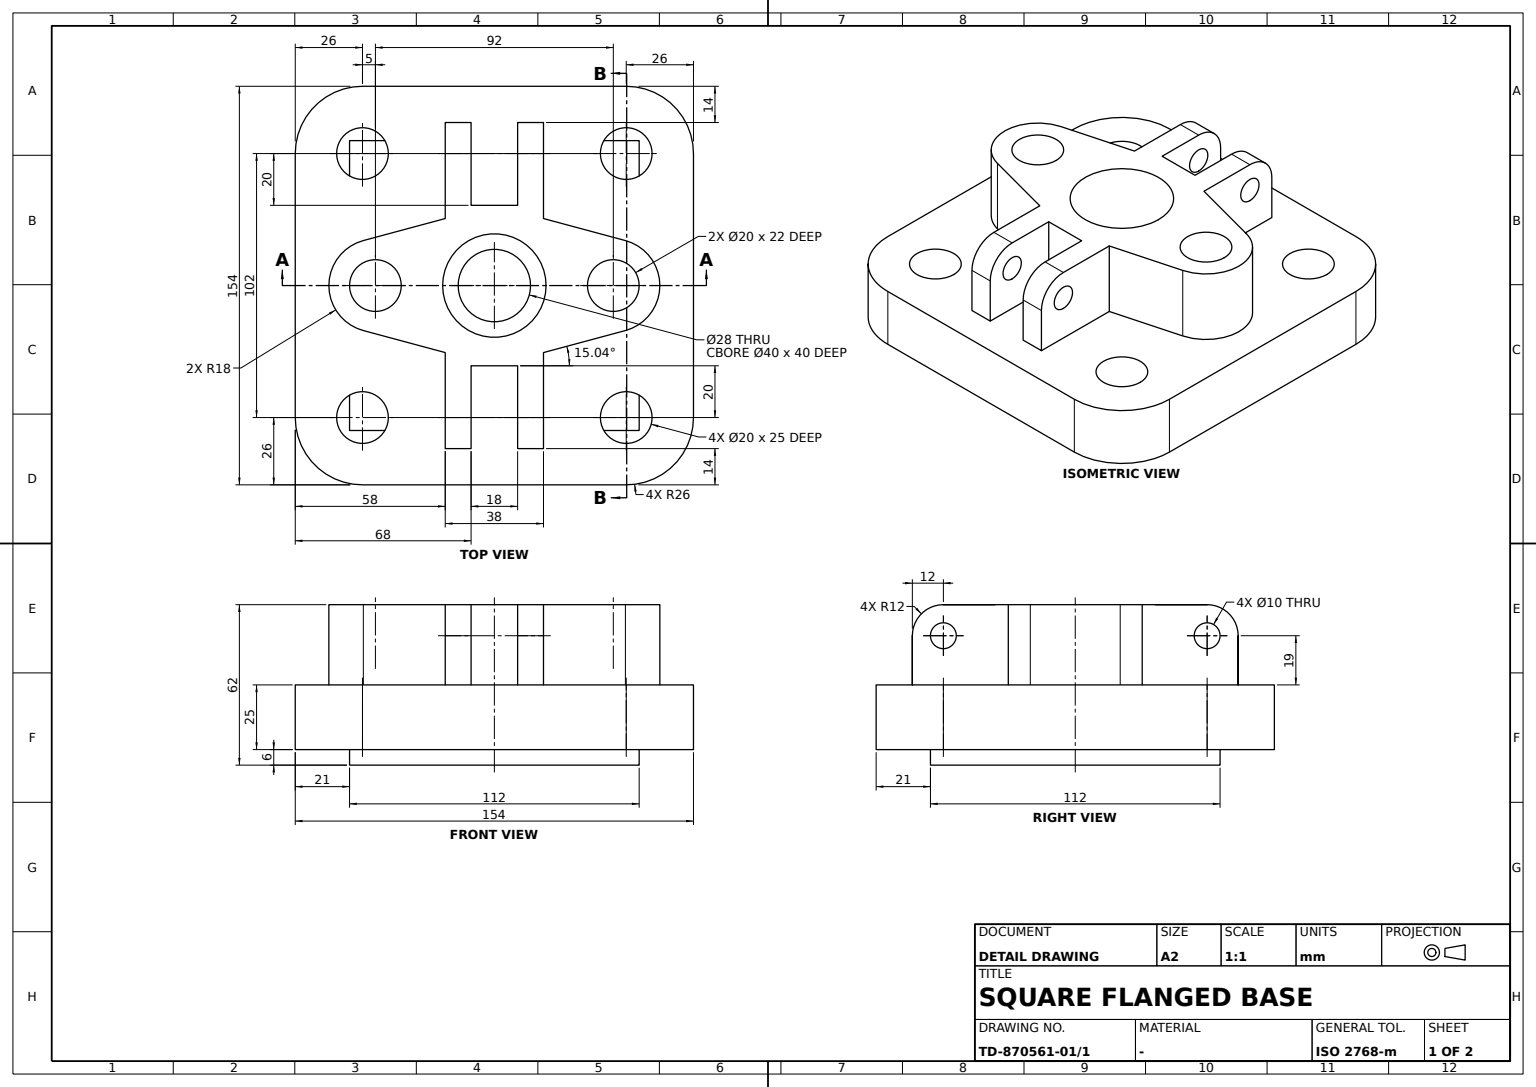
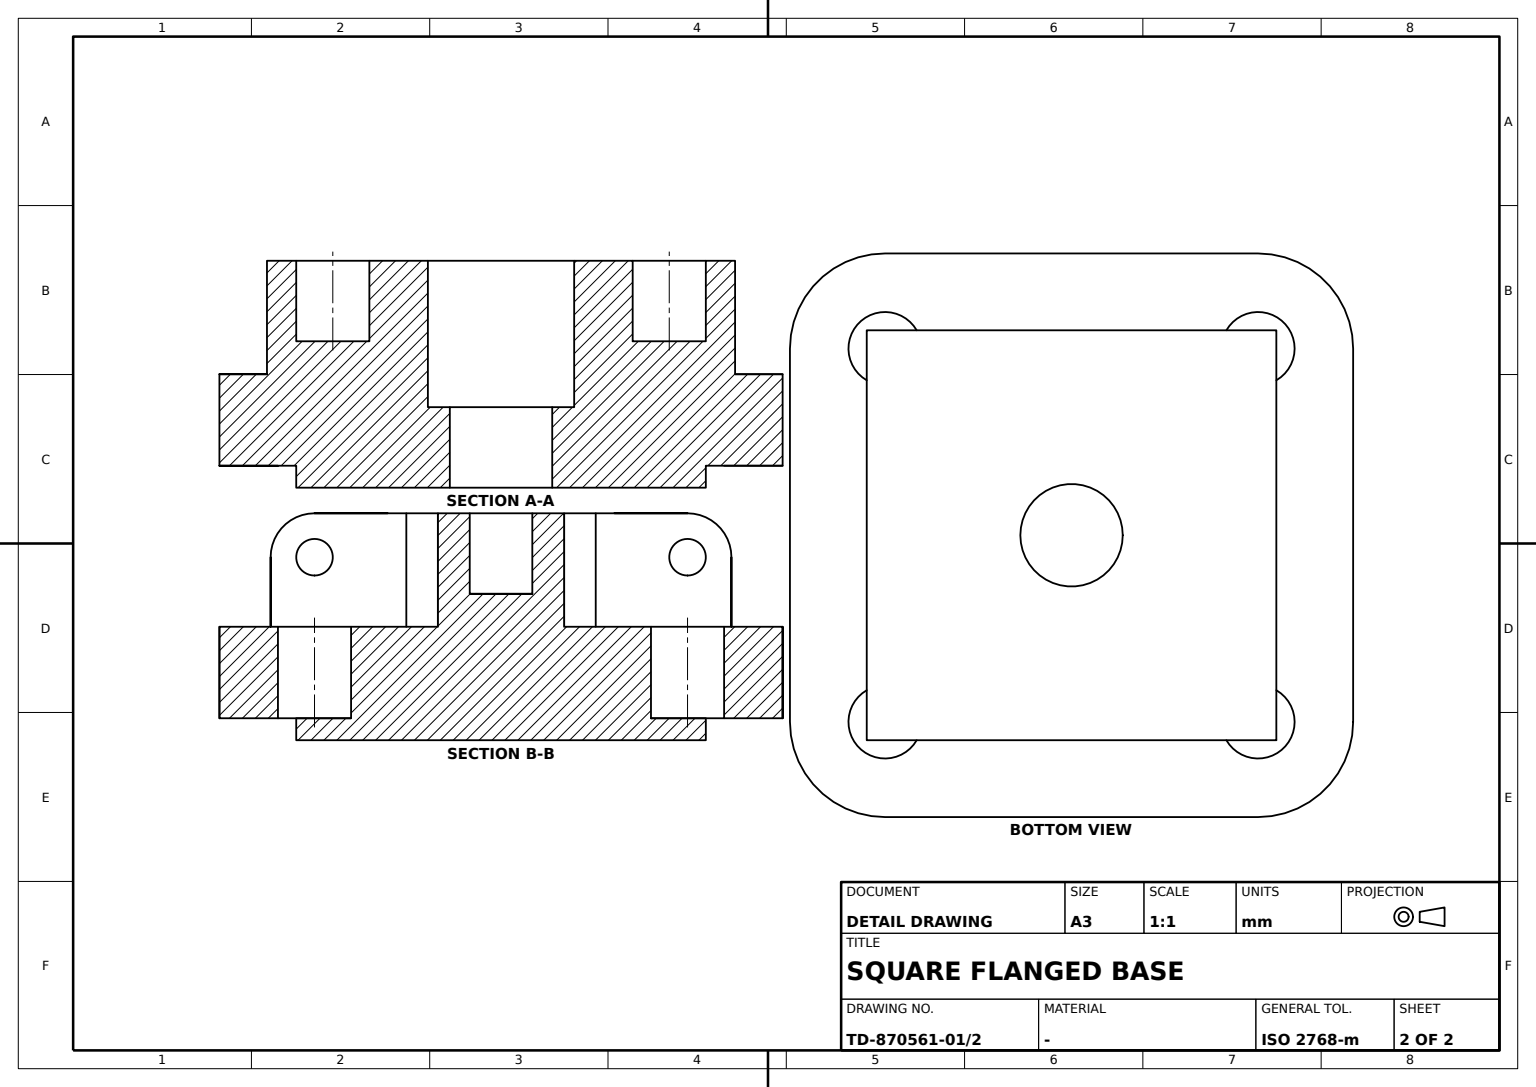
solid
v1 (-56,56,0)
v2 (-42.339746,56,0)
e1 v1 v2 LINE
v3 (-56,42.339746,0)
e2 v3 v1 LINE
e3 v3 v2 CIRCLE(AX(P(-51,51,0),D(0,0,1),D(1,0,0)),10)
face PLANE(AX(P(0,0,0),D(0,0,1),D(1,0,0))) [-e1 -e2 e3]
v4 (-56,-42.339746,0)
e4 v4 v3 LINE
v5 (-56,56,-6)
e5 v1 v5 LINE
v6 (-56,-56,-6)
e6 v6 v5 LINE
v7 (-56,-56,0)
e7 v7 v6 LINE
e8 v7 v4 LINE
face PLANE(AX(P(-56,-56,0),D(-1,0,0),D(0,1,0))) [e4 e2 e5 -e6 -e7 e8]
v8 (56,42.339746,0)
v9 (56,-42.339746,0)
e9 v8 v9 LINE
v10 (56,-56,0)
e10 v9 v10 LINE
v11 (56,-56,-6)
e11 v10 v11 LINE
v12 (56,56,-6)
e12 v12 v11 LINE
v13 (56,56,0)
e13 v13 v12 LINE
e14 v13 v8 LINE
face PLANE(AX(P(56,56,0),D(1,0,0),D(0,-1,0))) [e9 e10 e11 -e12 -e13 e14]
v14 (-36,0,34)
e15 v14 v14 CIRCLE(AX(P(-46,0,34),D(0,0,1),D(1,0,0)),10)
face PLANE(AX(P(0,0,34),D(0,0,1),D(1,0,0))) [e15]
v15 (19,63,44)
v16 (19,51,56)
e16 v15 v16 CIRCLE(AX(P(19,51,44),D(1,0,0),D(0,0,-1)),12)
v17 (9,63,44)
e17 v17 v15 LINE
v18 (9,51,56)
e18 v18 v17 CIRCLE(AX(P(9,51,44),D(-1,0,0),D(0,0,1)),12)
e19 v18 v16 LINE
face CYL(AX(P(0,51,44),D(1,0,0),D(0,1,0)),12) [-e16 -e17 -e18 e19]
v19 (9,-51,56)
v20 (19,-51,56)
e20 v19 v20 LINE
v21 (9,-63,44)
e21 v21 v19 CIRCLE(AX(P(9,-51,44),D(-1,0,0),D(0,0,1)),12)
v22 (19,-63,44)
e22 v21 v22 LINE
e23 v20 v22 CIRCLE(AX(P(19,-51,44),D(1,0,0),D(0,0,-1)),12)
face CYL(AX(P(0,-51,44),D(1,0,0),D(0,-1,0)),12) [-e20 -e21 e22 -e23]
v23 (50.671343,-17.383284,25)
v24 (50.671343,17.383284,25)
e24 v23 v24 CIRCLE(AX(P(46,0,25),D(0,0,1),D(1,0,0)),18)
v25 (50.671343,17.383284,56)
e25 v24 v25 LINE
v26 (50.671343,-17.383284,56)
e26 v26 v25 CIRCLE(AX(P(46,0,56),D(0,0,1),D(1,0,0)),18)
e27 v23 v26 LINE
face CYL(AX(P(46,0,28),D(0,0,1),D(1,0,0)),18) [e24 e25 -e26 -e27]
v27 (77,51,25)
v28 (51,77,25)
e28 v27 v28 CIRCLE(AX(P(51,51,25),D(0,0,1),D(1,0,0)),26)
v29 (-51,77,25)
e29 v29 v28 LINE
v30 (-77,51,25)
e30 v29 v30 CIRCLE(AX(P(-51,51,25),D(0,0,1),D(1,0,0)),26)
v31 (-77,-51,25)
e31 v31 v30 LINE
v32 (-51,-77,25)
e32 v31 v32 CIRCLE(AX(P(-51,-51,25),D(0,0,1),D(1,0,0)),26)
v33 (51,-77,25)
e33 v33 v32 LINE
v34 (77,-51,25)
e34 v33 v34 CIRCLE(AX(P(51,-51,25),D(0,0,1),D(1,0,0)),26)
e35 v27 v34 LINE
v35 (61,-51,25)
e36 v35 v35 CIRCLE(AX(P(51,-51,25),D(0,0,1),D(1,0,0)),10)
v36 (61,51,25)
e37 v36 v36 CIRCLE(AX(P(51,51,25),D(0,0,1),D(1,0,0)),10)
v37 (-41,-51,25)
e38 v37 v37 CIRCLE(AX(P(-51,-51,25),D(0,0,1),D(1,0,0)),10)
v38 (-41,51,25)
e39 v38 v38 CIRCLE(AX(P(-51,51,25),D(0,0,1),D(1,0,0)),10)
v39 (19,-63,25)
v40 (19,-25.894203,25)
e40 v39 v40 LINE
v41 (9,-63,25)
e41 v41 v39 LINE
v42 (9,-31,25)
e42 v42 v41 LINE
v43 (-9,-31,25)
e43 v43 v42 LINE
v44 (-9,-63,25)
e44 v44 v43 LINE
v45 (-19,-63,25)
e45 v45 v44 LINE
v46 (-19,-25.894203,25)
e46 v46 v45 LINE
v47 (-50.671343,-17.383284,25)
e47 v46 v47 LINE
v48 (-50.671343,17.383284,25)
e48 v48 v47 CIRCLE(AX(P(-46,0,25),D(0,0,1),D(1,0,0)),18)
v49 (-19,25.894203,25)
e49 v49 v48 LINE
v50 (-19,63,25)
e50 v50 v49 LINE
v51 (-9,63,25)
e51 v50 v51 LINE
v52 (-9,31,25)
e52 v52 v51 LINE
v53 (9,31,25)
e53 v52 v53 LINE
v54 (9,63,25)
e54 v54 v53 LINE
v55 (19,63,25)
e55 v54 v55 LINE
v56 (19,25.894203,25)
e56 v56 v55 LINE
e57 v56 v24 LINE
e58 v40 v23 LINE
face PLANE(AX(P(0,0,25),D(0,0,1),D(1,0,0))) [e28 -e29 e30 -e31 e32 -e33 e34 -e35] [-e36] [-e37] [-e38] [-e39] [-e40 -e41 -e42 -e43 -e44 -e45 -e46 e47 -e48 -e49 -e50 e51 -e52 e53 -e54 e55 -e56 e57 -e24 -e58]
v57 (-9,-51,39)
e59 v57 v57 CIRCLE(AX(P(-9,-51,44),D(1,0,0),D(0,0,-1)),5)
v58 (-9,-51,56)
v59 (-9,-63,44)
e60 v58 v59 CIRCLE(AX(P(-9,-51,44),D(1,0,0),D(0,0,-1)),12)
e61 v44 v59 LINE
v60 (-9,-31,56)
e62 v43 v60 LINE
e63 v58 v60 LINE
face PLANE(AX(P(-9,-63,0),D(1,0,0),D(0,1,0))) [-e59] [e60 -e61 e44 e62 -e63]
v61 (-9,51,39)
e64 v61 v61 CIRCLE(AX(P(-9,51,44),D(1,0,0),D(0,0,-1)),5)
v62 (-19,51,49)
e65 v62 v62 CIRCLE(AX(P(-19,51,44),D(-1,0,0),D(0,0,1)),5)
face CYL(AX(P(0,51,44),D(1,0,0),D(0,1,0)),5) rev [e64] [e65]
v63 (51,-77,0)
v64 (-51,-77,0)
e66 v63 v64 LINE
e67 v63 v33 LINE
e68 v64 v32 LINE
face PLANE(AX(P(51,-77,0),D(0,1,0),D(-1,0,0))) rev [-e66 e67 e33 -e68]
v65 (19,25.894203,56)
e69 v56 v65 LINE
e70 v65 v25 LINE
face PLANE(AX(P(19,25.894203,0),D(-0.259519075,-0.965737982,0),D(0.965737982,-0.259519075,0))) rev [e69 e70 -e25 -e57]
v66 (-19,-63,44)
e71 v66 v59 LINE
e72 v45 v66 LINE
face PLANE(AX(P(-19,-63,0),D(0,-1,0),D(1,0,0))) [e45 e61 -e71 -e72]
v67 (-9,63,44)
v68 (-9,51,56)
e73 v67 v68 CIRCLE(AX(P(-9,51,44),D(1,0,0),D(0,0,-1)),12)
v69 (-19,63,44)
e74 v69 v67 LINE
v70 (-19,51,56)
e75 v70 v69 CIRCLE(AX(P(-19,51,44),D(-1,0,0),D(0,0,1)),12)
e76 v70 v68 LINE
face CYL(AX(P(0,51,44),D(1,0,0),D(0,1,0)),12) [-e73 -e74 -e75 e76]
v71 (-19,-51,56)
e77 v71 v58 LINE
e78 v66 v71 CIRCLE(AX(P(-19,-51,44),D(-1,0,0),D(0,0,1)),12)
face CYL(AX(P(0,-51,44),D(1,0,0),D(0,-1,0)),12) [e71 -e60 -e77 -e78]
v72 (42.339746,-56,0)
e79 v10 v72 LINE
e80 v9 v72 CIRCLE(AX(P(51,-51,0),D(0,0,1),D(1,0,0)),10)
face PLANE(AX(P(0,0,0),D(0,0,1),D(1,0,0))) [-e79 -e10 e80]
e81 v50 v69 LINE
v73 (-19,25.894203,56)
e82 v49 v73 LINE
e83 v73 v70 LINE
face PLANE(AX(P(-19,-25.894203,0),D(-1,0,0),D(0,-1,0))) [-e81 e50 e82 e83 e75] [-e65]
e84 v54 v17 LINE
v74 (9,31,56)
e85 v53 v74 LINE
e86 v74 v18 LINE
v75 (9,51,49)
e87 v75 v75 CIRCLE(AX(P(9,51,44),D(-1,0,0),D(0,0,1)),5)
face PLANE(AX(P(9,-31,0),D(-1,0,0),D(0,-1,0))) [-e84 e54 e85 e86 e18] [-e87]
v76 (42.339746,56,0)
e88 v8 v76 CIRCLE(AX(P(51,51,0),D(0,0,1),D(1,0,0)),10)
e89 v76 v8 CIRCLE(AX(P(51,51,0),D(0,0,1),D(1,0,0)),10)
face CYL(AX(P(51,51,12.5),D(0,0,1),D(1,0,0)),10) rev [e37] [-e88 -e89]
e90 v51 v67 LINE
face PLANE(AX(P(9,63,0),D(0,-1,0),D(1,0,0))) rev [e74 -e90 -e51 e81]
e91 v76 v13 LINE
face PLANE(AX(P(0,0,0),D(0,0,1),D(1,0,0))) [-e14 -e91 e89]
v77 (56,0,34)
e92 v77 v77 CIRCLE(AX(P(46,0,34),D(0,0,1),D(1,0,0)),10)
face PLANE(AX(P(0,0,34),D(0,0,1),D(1,0,0))) [e92]
v78 (9,-51,49)
e93 v78 v78 CIRCLE(AX(P(9,-51,44),D(-1,0,0),D(0,0,1)),5)
e94 v41 v21 LINE
v79 (9,-31,56)
e95 v79 v19 LINE
e96 v42 v79 LINE
face PLANE(AX(P(9,-31,0),D(-1,0,0),D(0,-1,0))) [-e93] [e42 e94 e21 -e95 -e96]
v80 (-50.671343,17.383284,56)
e97 v48 v80 LINE
v81 (-50.671343,-17.383284,56)
e98 v47 v81 LINE
e99 v80 v81 CIRCLE(AX(P(-46,0,56),D(0,0,1),D(1,0,0)),18)
face CYL(AX(P(-46,0,28),D(0,0,1),D(1,0,0)),18) [-e97 e48 e98 -e99]
v82 (-51,77,0)
v83 (51,77,0)
e100 v82 v83 LINE
e101 v82 v29 LINE
e102 v83 v28 LINE
face PLANE(AX(P(-51,77,0),D(0,-1,0),D(1,0,0))) rev [-e100 e101 e29 -e102]
v84 (77,-51,0)
e103 v84 v34 LINE
v85 (77,51,0)
e104 v85 v84 LINE
e105 v85 v27 LINE
face PLANE(AX(P(77,51,0),D(-1,0,0),D(0,-1,0))) rev [e35 -e103 -e104 e105]
e106 v60 v79 LINE
face PLANE(AX(P(-9,-31,0),D(0,-1,0),D(1,0,0))) [e96 -e106 -e62 e43]
v86 (-36,0,56)
e107 v86 v86 CIRCLE(AX(P(-46,0,56),D(0,0,1),D(1,0,0)),10)
face CYL(AX(P(-46,0,45),D(0,0,1),D(1,0,0)),10) rev [-e15] [e107]
v87 (19,51,39)
e108 v87 v87 CIRCLE(AX(P(19,51,44),D(1,0,0),D(0,0,-1)),5)
e109 v55 v15 LINE
e110 v16 v65 LINE
face PLANE(AX(P(19,-63,0),D(1,0,0),D(0,1,0))) [-e108] [e109 e16 e110 -e69 e56]
v88 (-42.339746,-56,0)
e111 v88 v4 CIRCLE(AX(P(-51,-51,0),D(0,0,1),D(1,0,0)),10)
e112 v4 v88 CIRCLE(AX(P(-51,-51,0),D(0,0,1),D(1,0,0)),10)
face CYL(AX(P(-51,-51,12.5),D(0,0,1),D(1,0,0)),10) rev [-e111 -e112] [e38]
e113 v2 v3 CIRCLE(AX(P(-51,51,0),D(0,0,1),D(1,0,0)),10)
face CYL(AX(P(-51,51,12.5),D(0,0,1),D(1,0,0)),10) rev [-e3 -e113] [e39]
v89 (-77,-51,0)
e114 v89 v31 LINE
e115 v89 v64 CIRCLE(AX(P(-51,-51,0),D(0,0,1),D(1,0,0)),26)
face CYL(AX(P(-51,-51,12.5),D(0,0,1),D(1,0,0)),26) [-e114 e115 e68 -e32]
v90 (-19,-51,49)
e116 v90 v90 CIRCLE(AX(P(-19,-51,44),D(-1,0,0),D(0,0,1)),5)
v91 (-19,-25.894203,56)
e117 v91 v71 LINE
e118 v46 v91 LINE
face PLANE(AX(P(-19,-25.894203,0),D(-1,0,0),D(0,-1,0))) [-e116] [e46 e72 e78 -e117 -e118]
v92 (20,0,16)
e119 v92 v92 CIRCLE(AX(P(0,0,16),D(0,0,1),D(1,0,0)),20)
v93 (20,0,56)
e120 v93 v93 CIRCLE(AX(P(0,0,56),D(0,0,1),D(1,0,0)),20)
face CYL(AX(P(0,0,36),D(0,0,1),D(1,0,0)),20) rev [-e119] [e120]
v94 (-77,51,0)
e121 v94 v30 LINE
e122 v89 v94 LINE
face PLANE(AX(P(-77,-51,0),D(1,0,0),D(0,1,0))) rev [-e121 -e122 e114 e31]
e123 v91 v81 LINE
face PLANE(AX(P(-19,-25.894203,0),D(0.259519075,0.965737982,0),D(-0.965737982,0.259519075,0))) rev [-e98 -e47 e118 e123]
face CYL(AX(P(0,-51,44),D(1,0,0),D(0,1,0)),5) rev [e116] [e59]
e124 v85 v83 CIRCLE(AX(P(51,51,0),D(0,0,1),D(1,0,0)),26)
face CYL(AX(P(51,51,12.5),D(0,0,1),D(1,0,0)),26) [e102 -e28 -e105 e124]
v95 (14,0,16)
e125 v95 v95 CIRCLE(AX(P(0,0,16),D(0,0,1),D(1,0,0)),14)
v96 (14,0,-6)
e126 v96 v96 CIRCLE(AX(P(0,0,-6),D(0,0,1),D(1,0,0)),14)
face CYL(AX(P(0,0,36),D(0,0,1),D(1,0,0)),14) rev [e125] [-e126]
e127 v88 v7 LINE
e128 v11 v6 LINE
e129 v72 v88 LINE
face PLANE(AX(P(56,-56,0),D(0,-1,0),D(-1,0,0))) [e127 e7 -e128 -e11 e79 e129]
v97 (19,-25.894203,56)
e130 v40 v97 LINE
e131 v97 v26 LINE
face PLANE(AX(P(19,-25.894203,0),D(0.259519075,-0.965737982,0),D(0.965737982,0.259519075,0))) [-e130 e58 e27 -e131]
e132 v2 v76 LINE
e133 v5 v12 LINE
face PLANE(AX(P(-56,56,0),D(0,1,0),D(1,0,0))) [-e5 e1 e132 e91 e13 -e133]
v98 (56,0,56)
e134 v98 v98 CIRCLE(AX(P(46,0,56),D(0,0,1),D(1,0,0)),10)
face CYL(AX(P(46,0,45),D(0,0,1),D(1,0,0)),10) rev [-e92] [e134]
e135 v82 v94 CIRCLE(AX(P(-51,51,0),D(0,0,1),D(1,0,0)),26)
face CYL(AX(P(-51,51,12.5),D(0,0,1),D(1,0,0)),26) [e135 e121 -e30 -e101]
face PLANE(AX(P(9,63,0),D(0,-1,0),D(1,0,0))) rev [e84 e17 -e109 -e55]
v99 (-9,31,56)
e136 v52 v99 LINE
e137 v99 v74 LINE
face PLANE(AX(P(-9,31,0),D(0,-1,0),D(1,0,0))) rev [-e53 e136 e137 -e85]
face CYL(AX(P(0,51,44),D(1,0,0),D(0,1,0)),5) rev [e87] [e108]
face PLANE(AX(P(0,0,0),D(0,0,1),D(1,0,0))) [-e8 -e127 e111]
face PLANE(AX(P(0,0,16),D(0,0,1),D(1,0,0))) [e119] [-e125]
e138 v39 v22 LINE
e139 v20 v97 LINE
v100 (19,-51,39)
e140 v100 v100 CIRCLE(AX(P(19,-51,44),D(1,0,0),D(0,0,-1)),5)
face PLANE(AX(P(19,-63,0),D(1,0,0),D(0,1,0))) [e23 -e138 e40 e130 -e139] [-e140]
e141 v72 v9 CIRCLE(AX(P(51,-51,0),D(0,0,1),D(1,0,0)),10)
face CYL(AX(P(51,-51,12.5),D(0,0,1),D(1,0,0)),10) rev [e36] [-e80 -e141]
e142 v63 v84 CIRCLE(AX(P(51,-51,0),D(0,0,1),D(1,0,0)),26)
face PLANE(AX(P(0,0,0),D(0,0,1),D(1,0,0))) rev [e88 -e132 e113 -e4 e112 -e129 e141 -e9] [-e115 e122 -e135 e100 -e124 e104 -e142 e66]
face CYL(AX(P(0,-51,44),D(1,0,0),D(0,1,0)),5) rev [e140] [e93]
face PLANE(AX(P(0,0,-6),D(0,0,1),D(1,0,0))) rev [e133 e12 e128 e6] [e126]
e143 v73 v80 LINE
face PLANE(AX(P(-19,25.894203,0),D(-0.259519075,0.965737982,0),D(-0.965737982,-0.259519075,0))) [e97 -e143 -e82 e49]
e144 v68 v99 LINE
face PLANE(AX(P(-9,-63,0),D(1,0,0),D(0,1,0))) [-e64] [-e136 e52 e90 e73 e144]
face PLANE(AX(P(-19,-63,0),D(0,-1,0),D(1,0,0))) [e41 e138 -e22 -e94]
face PLANE(AX(P(0,0,56),D(0,0,1),D(1,0,0))) [e26 -e70 -e110 -e19 -e86 -e137 -e144 -e76 -e83 e143 e99 -e123 e117 e77 e63 e106 e95 e20 e139 e131] [-e134] [-e107] [-e120]
face CYL(AX(P(51,-51,12.5),D(0,0,1),D(1,0,0)),26) [e103 -e34 -e67 e142]
